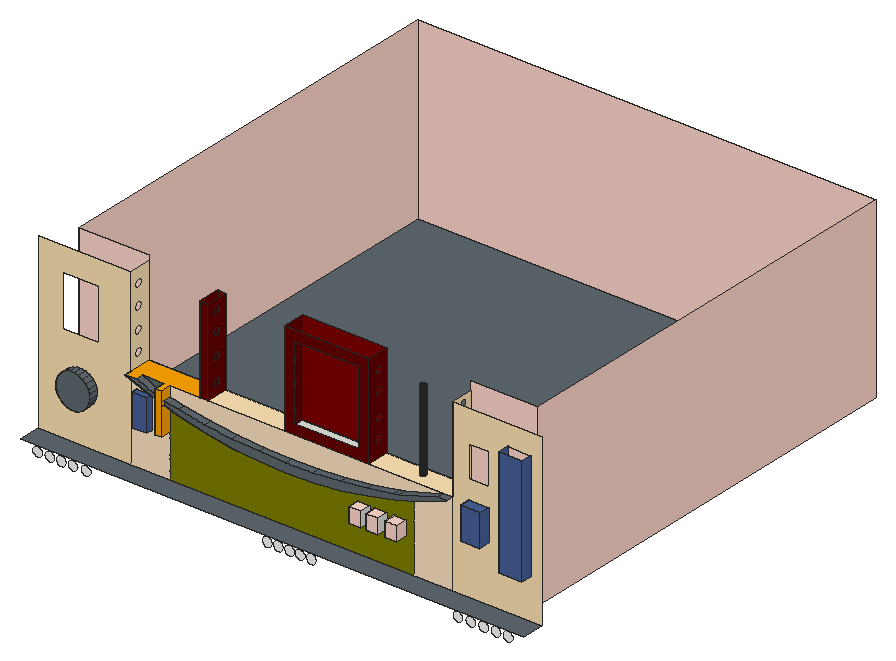
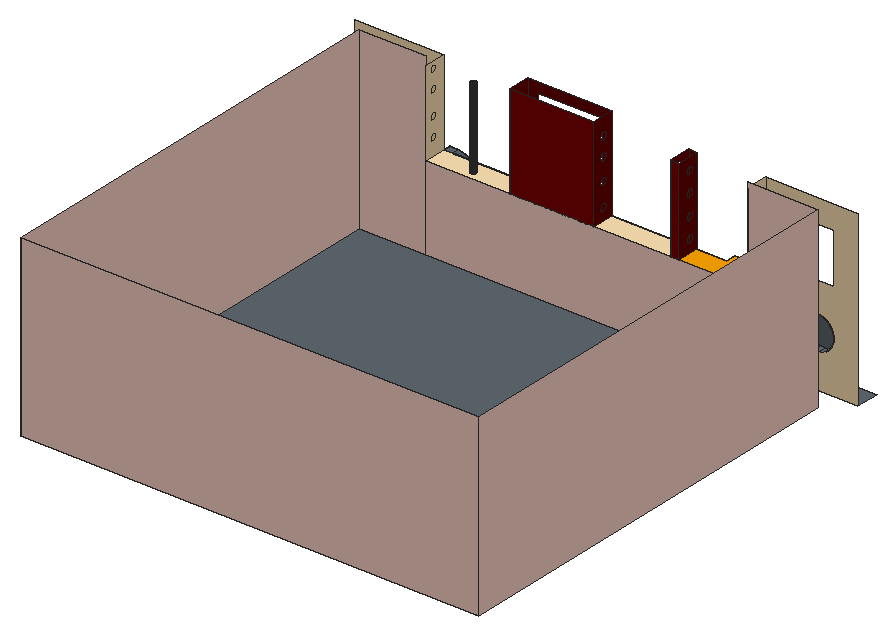
# SketchUp Ruby script. Lengths in inches.
U = 1.inch
M = Sketchup.active_model
def pt(a) = Geom::Point3d.new(a.map { |v| v * U })
def face(e, loops, mat)
  f = e.add_face(loops[0].map { |a| pt(a) })
  loops[1..].each { |l| e.add_face(l.map { |a| pt(a) }).erase! }
  f.material = f.back_material = mat if mat
  f
end
# faces: each face lists its corners as indices into pts; further lists are holes
def faces(e, pts, list, mat = nil) = list.each { |f| face(e, (f[0].is_a?(Array) ? f : [f]).map { |l| l.map { |i| pts[i] } }, mat) }
# xy, xz, yz: faces in a plane at the given z, y or x. An outline is a flat list of corners, or four numbers for a rectangle; further outlines are holes
def ring(l) = l.size == 4 ? [[l[0], l[1]], [l[2], l[1]], [l[2], l[3]], [l[0], l[3]]] : l.each_slice(2).to_a
def flat(e, list, mat, &to3) = list.each { |f| face(e, (f[0].is_a?(Array) ? f : [f]).map { |l| ring(l).map { |u, v| to3.(u, v) } }, mat) }
def xy(e, z, list, mat = nil) = flat(e, list, mat) { |x, y| [x, y, z] }
def xz(e, y, list, mat = nil) = flat(e, list, mat) { |x, z| [x, y, z] }
def yz(e, x, list, mat = nil) = flat(e, list, mat) { |y, z| [x, y, z] }
def lines(e, pts, list) = list.each { |a, b| e.add_line(pt(pts[a]), pt(pts[b])) }
# prism: a flat outline (further loops are holes) pulled along v
def prism(e, loops, v, mat = nil)
  f = face(e, loops, mat); d = Geom::Vector3d.new(v.map { |x| x * U })
  f.pushpull(f.normal.samedirection?(d) ? d.length : -d.length)
end
def box(e, o, s, mat = nil) = prism(e, [[o, [o[0] + s[0], o[1], o[2]], [o[0] + s[0], o[1] + s[1], o[2]], [o[0], o[1] + s[1], o[2]]]], [0, 0, s[2]], mat)
def at(x, y, z, deg = 0) = Geom::Transformation.translation(pt([x, y, z])) * Geom::Transformation.rotation(ORIGIN, Z_AXIS, deg.degrees)
def axes(o, x, y, z) = Geom::Transformation.new([*x, 0, *y, 0, *z, 0, *pt(o).to_a, 1])
def part(name) = M.definitions.add(name)
# library, detail: a bought-in or finely detailed component or shape, given as its bounding box
def library(name, o, s) = part(name).tap { |d| box(d.entities, o, s) }
def detail(e, o, s) = box(e.add_group.entities, o, s)
def put(e, d, t, mat = nil) = e.add_instance(d, t).tap { |i| i.material = mat if mat }
def group(e, t, mat = nil) = e.add_group.tap { |g| g.transformation = t; g.material = mat if mat }.entities
root = M.entities
M.materials.add("[0012_Bisque]").color = [255, 228, 196]
M.materials.add("[0022_Maroon]").color = [128, 0, 0]
M.materials.add("[0032_Moccasin]").color = [255, 228, 181]
M.materials.add("[0038_Orange]").color = [255, 165, 0]
M.materials.add("[0058_Olive]").color = [128, 128, 0]
M.materials.add("[Color A08]").color = [102, 0, 0]
M.materials.add("[Color B01]").color = [255, 216, 204]
M.materials.add("[Color M07]").color = [58, 58, 58]
M.materials.add("[Formica Blue]").color = [71, 97, 152]
M.materials.add("[Formica Speckled Grey]").color = [94, 105, 111]
M.materials.add("[Quartz Light Grey]").color = [251, 251, 252]
xy(root,133.625,[[47,20.01,251.02,29.17],[56.16,38.27,241.86,209.77]],"[Formica Speckled Grey]")
xy(root,146.7,[[176.27,24.54,181.08,29.17],[183.39,24.54,188.2,29.17],[191.08,24.54,195.89,29.17]],"[Color B01]")
xy(root,148.88,[[86.87,26.79,92.74,29.17]],"[Formica Blue]")
xy(root,149.75,[[236.96,24.73,246.46,29.17]],"[Formica Blue]")
xy(root,151.0625,[[97.68,24.86,100.35,29.17]],"[0038_Orange]")
xy(root,152.64,[[176.27,24.54,181.08,29.17],[183.39,24.54,188.2,29.17],[191.08,24.54,195.89,29.17]],"[Color B01]")
xy(root,155.96,[[221.42,24.73,229.42,29.17]],"[Formica Blue]")
xy(root,161.88,[[86.87,26.79,92.74,29.17]],"[Formica Blue]")
xy(root,167.625,[[112.25,29.17,115.75,38.27],[146.64,29.17,180.76,38.27]])
xy(root,167.625,[[115.75,29.17,146.64,38.27],[[180.76,29.17,214.88,38.27],[198.48,33.52,198.21,33.56,197.95,33.66,197.73,33.83,197.5625,34.05,197.46,34.31,197.42,34.58,197.46,34.86,197.5625,35.12,197.73,35.34,197.95,35.5,198.21,35.61,198.48,35.65,198.76,35.61,199.01,35.5,199.23,35.34,199.4,35.12,199.51,34.86,199.55,34.58,199.51,34.31,199.4,34.05,199.23,33.83,199.01,33.66,198.76,33.56]]],"[0032_Moccasin]")
xy(root,167.625,[[97.68,24.86,100.35,24.86,100.35,29.17,112.25,29.17,112.25,38.27,84.58,38.27,84.58,26.11,89.25,26.11,89.25,29.17,97.68,29.17]],"[0038_Orange]")
xy(root,167.625,[[211.24,26.11,214.88,29.17]],"[Formica Speckled Grey]")
xy(root,168.9,[[221.42,24.73,229.42,29.17]],"[Formica Blue]")
xz(root,20.01,[[54,129.67,54.47,129.73,54.9,129.91,55.28,130.2,55.57,130.57,55.75,131.01,55.81,131.48,55.75,131.95,55.57,132.38,55.28,132.76,54.9,133.05,54.47,133.23,54,133.29,53.53,133.23,53.09,133.05,52.72,132.76,52.43,132.38,52.25,131.95,52.19,131.48,52.25,131.01,52.43,130.57,52.72,130.2,53.09,129.91,53.53,129.73],[58.94,129.67,59.4,129.73,59.84,129.91,60.22,130.2,60.5,130.57,60.6875,131.01,60.75,131.48,60.6875,131.95,60.5,132.38,60.22,132.76,59.84,133.05,59.4,133.23,58.94,133.29,58.47,133.23,58.03,133.05,57.65,132.76,57.37,132.38,57.18,131.95,57.12,131.48,57.18,131.01,57.37,130.57,57.65,130.2,58.03,129.91,58.47,129.73],[63.56,129.67,64.03,129.73,64.47,129.91,64.84,130.2,65.13,130.57,65.3125,131.01,65.37,131.48,65.3125,131.95,65.13,132.38,64.84,132.76,64.47,133.05,64.03,133.23,63.56,133.29,63.09,133.23,62.65,133.05,62.28,132.76,61.99,132.38,61.81,131.95,61.75,131.48,61.81,131.01,61.99,130.57,62.28,130.2,62.65,129.91,63.09,129.73],[68.31,129.67,68.78,129.73,69.22,129.91,69.59,130.2,69.88,130.57,70.0625,131.01,70.12,131.48,70.0625,131.95,69.88,132.38,69.59,132.76,69.22,133.05,68.78,133.23,68.31,133.29,67.84,133.23,67.4,133.05,67.03,132.76,66.74,132.38,66.56,131.95,66.5,131.48,66.56,131.01,66.74,130.57,67.03,130.2,67.4,129.91,67.84,129.73],[73.62,129.67,74.09,129.73,74.53,129.91,74.9,130.2,75.19,130.57,75.375,131.01,75.44,131.48,75.375,131.95,75.19,132.38,74.9,132.76,74.53,133.05,74.09,133.23,73.62,133.29,73.15,133.23,72.72,133.05,72.34,132.76,72.05,132.38,71.87,131.95,71.81,131.48,71.87,131.01,72.05,130.57,72.34,130.2,72.72,129.91,73.15,129.73],
  [147.06,129.67,147.53,129.73,147.97,129.91,148.34,130.2,148.63,130.57,148.8125,131.01,148.87,131.48,148.8125,131.95,148.63,132.38,148.34,132.76,147.97,133.05,147.53,133.23,147.06,133.29,146.59,133.23,146.15,133.05,145.78,132.76,145.49,132.38,145.31,131.95,145.25,131.48,145.31,131.01,145.49,130.57,145.78,130.2,146.15,129.91,146.59,129.73],[151.44,129.67,151.9,129.73,152.34,129.91,152.72,130.2,153,130.57,153.1875,131.01,153.25,131.48,153.1875,131.95,153,132.38,152.72,132.76,152.34,133.05,151.9,133.23,151.44,133.29,150.97,133.23,150.53,133.05,150.15,132.76,149.87,132.38,149.68,131.95,149.62,131.48,149.68,131.01,149.87,130.57,150.15,130.2,150.53,129.91,150.97,129.73],[156,129.67,156.47,129.73,156.9,129.91,157.28,130.2,157.57,130.57,157.75,131.01,157.81,131.48,157.75,131.95,157.57,132.38,157.28,132.76,156.9,133.05,156.47,133.23,156,133.29,155.53,133.23,155.09,133.05,154.72,132.76,154.43,132.38,154.25,131.95,154.19,131.48,154.25,131.01,154.43,130.57,154.72,130.2,155.09,129.91,155.53,129.73],[160.31,129.67,160.78,129.73,161.22,129.91,161.59,130.2,161.88,130.57,162.0625,131.01,162.12,131.48,162.0625,131.95,161.88,132.38,161.59,132.76,161.22,133.05,160.78,133.23,160.31,133.29,159.84,133.23,159.4,133.05,159.03,132.76,158.74,132.38,158.56,131.95,158.5,131.48,158.56,131.01,158.74,130.57,159.03,130.2,159.4,129.91,159.84,129.73],[164.87,129.67,165.34,129.73,165.78,129.91,166.15,130.2,166.44,130.57,166.625,131.01,166.69,131.48,166.625,131.95,166.44,132.38,166.15,132.76,165.78,133.05,165.34,133.23,164.87,133.29,164.4,133.23,163.97,133.05,163.59,132.76,163.3,132.38,163.12,131.95,163.06,131.48,163.12,131.01,163.3,130.57,163.59,130.2,163.97,129.91,164.4,129.73],
  [224.19,129.67,224.65,129.73,225.09,129.91,225.47,130.2,225.75,130.57,225.9375,131.01,226,131.48,225.9375,131.95,225.75,132.38,225.47,132.76,225.09,133.05,224.65,133.23,224.19,133.29,223.72,133.23,223.28,133.05,222.9,132.76,222.62,132.38,222.43,131.95,222.37,131.48,222.43,131.01,222.62,130.57,222.9,130.2,223.28,129.91,223.72,129.73],[229.44,129.67,229.9,129.73,230.34,129.91,230.72,130.2,231,130.57,231.1875,131.01,231.25,131.48,231.1875,131.95,231,132.38,230.72,132.76,230.34,133.05,229.9,133.23,229.44,133.29,228.97,133.23,228.53,133.05,228.15,132.76,227.87,132.38,227.68,131.95,227.62,131.48,227.68,131.01,227.87,130.57,228.15,130.2,228.53,129.91,228.97,129.73],[234.56,129.67,235.03,129.73,235.47,129.91,235.84,130.2,236.13,130.57,236.3125,131.01,236.37,131.48,236.3125,131.95,236.13,132.38,235.84,132.76,235.47,133.05,235.03,133.23,234.56,133.29,234.09,133.23,233.65,133.05,233.28,132.76,232.99,132.38,232.81,131.95,232.75,131.48,232.81,131.01,232.99,130.57,233.28,130.2,233.65,129.91,234.09,129.73],[239.62,129.67,240.09,129.73,240.53,129.91,240.9,130.2,241.19,130.57,241.375,131.01,241.44,131.48,241.375,131.95,241.19,132.38,240.9,132.76,240.53,133.05,240.09,133.23,239.62,133.29,239.15,133.23,238.72,133.05,238.34,132.76,238.05,132.38,237.87,131.95,237.81,131.48,237.87,131.01,238.05,130.57,238.34,130.2,238.72,129.91,239.15,129.73],[244.56,129.67,245.03,129.73,245.47,129.91,245.84,130.2,246.13,130.57,246.3125,131.01,246.37,131.48,246.3125,131.95,246.13,132.38,245.84,132.76,245.47,133.05,245.03,133.23,244.56,133.29,244.09,133.23,243.65,133.05,243.28,132.76,242.99,132.38,242.81,131.95,242.75,131.48,242.81,131.01,242.99,130.57,243.28,130.2,243.65,129.91,244.09,129.73]],"[Quartz Light Grey]")
xz(root,24.54,[[176.27,146.7,181.08,152.64],[183.39,146.7,188.2,152.64],[191.08,146.7,195.89,152.64]],"[Color B01]")
xz(root,24.73,[[236.96,149.75,246.46,193.75],[221.42,155.96,229.42,168.9]],"[Formica Blue]")
xz(root,24.86,[[97.68,151.0625,100.35,167.625]],"[0038_Orange]")
xz(root,25.54,[[63.21,147.56,65.04,147.63,66.78,148.17,68.33,149.14,69.57,150.48,70.42,152.1,70.83,153.88,70.76,155.7,70.22,157.45,69.25,159,67.91,160.24,66.29,161.09,64.51,161.5,62.68,161.43,60.9375,160.89,59.39,159.92,58.15,158.57,57.29,156.96,56.89,155.18,56.96,153.35,57.5,151.61,58.47,150.06,59.8125,148.82,61.43,147.96]],"[Formica Speckled Grey]")
xz(root,26.11,[[149.73,154.76,160.86,155.12,171.95,156.2,182.9375,158,193.79,160.52,199.12,162.12,204.45,163.73,214.88,167.625,211.24,167.625,195.42,163.01,193.47,162.6,182.62,160.83,171.7,159.57,160.73,158.81,149.73,158.55,138.74,158.81,127.77,159.57,116.84,160.83,105.99,162.6,100.35,163.79,100.35,162.12,105.68,160.52,116.53,158,127.52,156.2,138.6,155.12],[97.68,162.92,97.68,164.35,96.14,164.67,89.25,167.625,84.58,167.625,95.02,163.73]],"[Formica Speckled Grey]")
xz(root,26.79,[[86.87,148.88,92.74,161.88]],"[Formica Blue]")
xz(root,29.17,[[[84.58,133.625,100.35,133.625,100.35,151.0625,97.68,151.0625,97.68,162.92,95.02,163.73,84.58,167.625],[86.87,148.88,92.74,161.88]],[199.12,133.625,214.88,133.625,214.88,167.625,204.45,163.73,199.12,162.12],[149.73,158.55,160.73,158.81,171.7,159.57,182.62,160.83,193.47,162.6,195.42,163.01,211.24,167.625,100.35,167.625,100.35,163.79,105.99,162.6,116.84,160.83,127.77,159.57,138.74,158.81]],"[0012_Bisque]")
xz(root,29.17,[[[47,133.625,84.58,203.49],[56.92,173.26,71.36,193.95],[63.21,147.56,61.43,147.96,59.8125,148.82,58.47,150.06,57.5,151.61,56.96,153.35,56.89,155.18,57.29,156.96,58.15,158.57,59.39,159.92,60.9375,160.89,62.68,161.43,64.51,161.5,66.29,161.09,67.91,160.24,69.25,159,70.22,157.45,70.76,155.7,70.83,153.88,70.42,152.1,69.57,150.48,68.33,149.14,66.78,148.17,65.04,147.63]],[[214.88,133.625,251.02,202.04],[236.96,149.75,246.46,193.75],[221.42,176.39,229.42,189.34],[221.42,155.96,229.42,168.9]]],"[0032_Moccasin]")
xz(root,29.17,[[[100.35,133.625,199.12,133.625,199.12,162.12,193.79,160.52,182.9375,158,171.95,156.2,160.86,155.12,149.73,154.76,138.6,155.12,127.52,156.2,116.53,158,105.68,160.52,100.35,162.12],[191.08,146.7,195.89,152.64],[183.39,146.7,188.2,152.64],[176.27,146.7,181.08,152.64]]],"[0058_Olive]")
xz(root,29.17,[[112.25,167.625,115.75,202.625],[[146.64,167.625,180.76,205.625],[150.55,171.54,176.84,201.71]]],"[Color A08]")
xz(root,29.17,[[97.68,164.35,97.68,167.625,89.25,167.625,96.14,164.67]],"[Formica Speckled Grey]")
xz(root,38.27,[[112.25,167.625,115.75,202.625],[146.64,167.625,180.76,205.625]],"[0022_Maroon]")
xz(root,38.27,[[56.16,133.625,84.58,205.625],[84.58,133.625,214.88,167.625],[214.88,133.625,241.86,205.625]],"[Color B01]")
xz(root,209.77,[[56.16,133.625,241.86,205.625]],"[Color B01]")
yz(root,56.16,[[38.27,133.625,209.77,205.625]],"[Color B01]")
yz(root,84.58,[[[29.17,167.625,38.27,203.49],[32.81,171.26,32.39,171.3125,32,171.47,31.66,171.73,31.4,172.07,31.24,172.46,31.18,172.88,31.24,173.3,31.4,173.69,31.66,174.03,32,174.29,32.39,174.45,32.81,174.51,33.23,174.45,33.62,174.29,33.96,174.03,34.22,173.69,34.38,173.3,34.43,172.88,34.38,172.46,34.22,172.07,33.96,171.73,33.62,171.47,33.23,171.3125],[32.81,179.38,32.39,179.4375,32,179.6,31.66,179.86,31.4,180.19,31.24,180.59,31.18,181.01,31.24,181.43,31.4,181.82,31.66,182.16,32,182.41,32.39,182.58,32.81,182.63,33.23,182.58,33.62,182.41,33.96,182.16,34.22,181.82,34.38,181.43,34.43,181.01,34.38,180.59,34.22,180.19,33.96,179.86,33.62,179.6,33.23,179.4375],[32.81,188.01,32.39,188.0625,32,188.22,31.66,188.48,31.4,188.82,31.24,189.21,31.18,189.63,31.24,190.05,31.4,190.44,31.66,190.78,32,191.04,32.39,191.2,32.81,191.26,33.23,191.2,33.62,191.04,33.96,190.78,34.22,190.44,34.38,190.05,34.43,189.63,34.38,189.21,34.22,188.82,33.96,188.48,33.62,188.22,33.23,188.0625],[32.81,196.19,32.39,196.25,32,196.41,31.66,196.67,31.4,197.01,31.24,197.4,31.18,197.82,31.24,198.24,31.4,198.63,31.66,198.97,32,199.23,32.39,199.39,32.81,199.44,33.23,199.39,33.62,199.23,33.96,198.97,34.22,198.63,34.38,198.24,34.43,197.82,34.38,197.4,34.22,197.01,33.96,196.67,33.62,196.41,33.23,196.25]]],"[0032_Moccasin]")
yz(root,86.87,[[26.79,148.88,29.17,161.88]],"[Formica Blue]")
yz(root,92.74,[[26.79,148.88,29.17,161.88]],"[Formica Blue]")
yz(root,97.68,[[24.86,151.0625,29.17,162.92],[24.86,162.92,26.11,164.35],[24.86,164.35,29.17,167.625]],"[0038_Orange]")
yz(root,100.35,[[24.86,151.0625,29.17,162.12],[24.86,162.12,26.11,163.79],[24.86,163.79,29.17,167.625]],"[0038_Orange]")
yz(root,112.25,[[[29.17,167.625,38.27,202.625],[32.81,196.19,33.23,196.25,33.62,196.41,33.96,196.67,34.22,197.01,34.38,197.4,34.43,197.82,34.38,198.24,34.22,198.63,33.96,198.97,33.62,199.23,33.23,199.39,32.81,199.44,32.39,199.39,32,199.23,31.66,198.97,31.4,198.63,31.24,198.24,31.18,197.82,31.24,197.4,31.4,197.01,31.66,196.67,32,196.41,32.39,196.25],[32.81,171.26,33.23,171.3125,33.62,171.47,33.96,171.73,34.22,172.07,34.38,172.46,34.43,172.88,34.38,173.3,34.22,173.69,33.96,174.03,33.62,174.29,33.23,174.45,32.81,174.51,32.39,174.45,32,174.29,31.66,174.03,31.4,173.69,31.24,173.3,31.18,172.88,31.24,172.46,31.4,172.07,31.66,171.73,32,171.47,32.39,171.3125],[32.81,188.01,33.23,188.0625,33.62,188.22,33.96,188.48,34.22,188.82,34.38,189.21,34.43,189.63,34.38,190.05,34.22,190.44,33.96,190.78,33.62,191.04,33.23,191.2,32.81,191.26,32.39,191.2,32,191.04,31.66,190.78,31.4,190.44,31.24,190.05,31.18,189.63,31.24,189.21,31.4,188.82,31.66,188.48,32,188.22,32.39,188.0625],[32.81,179.38,33.23,179.4375,33.62,179.6,33.96,179.86,34.22,180.19,34.38,180.59,34.43,181.01,34.38,181.43,34.22,181.82,33.96,182.16,33.62,182.41,33.23,182.58,32.81,182.63,32.39,182.58,32,182.41,31.66,182.16,31.4,181.82,31.24,181.43,31.18,181.01,31.24,180.59,31.4,180.19,31.66,179.86,32,179.6,32.39,179.4375]]],"[Color A08]")
yz(root,115.75,[[[29.17,167.625,38.27,202.625],[33.57,196.94,33.15,197,32.76,197.16,32.42,197.42,32.17,197.76,32,198.15,31.95,198.57,32,198.99,32.17,199.38,32.42,199.72,32.76,199.98,33.15,200.14,33.57,200.19,33.99,200.14,34.39,199.98,34.72,199.72,34.98,199.38,35.14,198.99,35.2,198.57,35.14,198.15,34.98,197.76,34.72,197.42,34.39,197.16,33.99,197],[33.57,170.94,33.15,171,32.76,171.16,32.42,171.42,32.17,171.76,32,172.15,31.95,172.57,32,172.99,32.17,173.38,32.42,173.72,32.76,173.98,33.15,174.14,33.57,174.19,33.99,174.14,34.39,173.98,34.72,173.72,34.98,173.38,35.14,172.99,35.2,172.57,35.14,172.15,34.98,171.76,34.72,171.42,34.39,171.16,33.99,171],[33.57,189.26,33.15,189.3125,32.76,189.47,32.42,189.73,32.17,190.07,32,190.46,31.95,190.88,32,191.3,32.17,191.69,32.42,192.03,32.76,192.29,33.15,192.45,33.57,192.51,33.99,192.45,34.39,192.29,34.72,192.03,34.98,191.69,35.14,191.3,35.2,190.88,35.14,190.46,34.98,190.07,34.72,189.73,34.39,189.47,33.99,189.3125],[33.57,180.44,33.15,180.5,32.76,180.66,32.42,180.92,32.17,181.26,32,181.65,31.95,182.07,32,182.49,32.17,182.88,32.42,183.22,32.76,183.48,33.15,183.64,33.57,183.69,33.99,183.64,34.39,183.48,34.72,183.22,34.98,182.88,35.14,182.49,35.2,182.07,35.14,181.65,34.98,181.26,34.72,180.92,34.39,180.66,33.99,180.5]]],"[Color A08]")
yz(root,146.64,[[[29.17,167.625,38.27,205.625],[33.57,196.94,33.99,197,34.39,197.16,34.72,197.42,34.98,197.76,35.14,198.15,35.2,198.57,35.14,198.99,34.98,199.38,34.72,199.72,34.39,199.98,33.99,200.14,33.57,200.19,33.15,200.14,32.76,199.98,32.42,199.72,32.17,199.38,32,198.99,31.95,198.57,32,198.15,32.17,197.76,32.42,197.42,32.76,197.16,33.15,197],[33.57,189.26,33.99,189.3125,34.39,189.47,34.72,189.73,34.98,190.07,35.14,190.46,35.2,190.88,35.14,191.3,34.98,191.69,34.72,192.03,34.39,192.29,33.99,192.45,33.57,192.51,33.15,192.45,32.76,192.29,32.42,192.03,32.17,191.69,32,191.3,31.95,190.88,32,190.46,32.17,190.07,32.42,189.73,32.76,189.47,33.15,189.3125],[33.57,180.44,33.99,180.5,34.39,180.66,34.72,180.92,34.98,181.26,35.14,181.65,35.2,182.07,35.14,182.49,34.98,182.88,34.72,183.22,34.39,183.48,33.99,183.64,33.57,183.69,33.15,183.64,32.76,183.48,32.42,183.22,32.17,182.88,32,182.49,31.95,182.07,32,181.65,32.17,181.26,32.42,180.92,32.76,180.66,33.15,180.5],[33.57,170.94,33.99,171,34.39,171.16,34.72,171.42,34.98,171.76,35.14,172.15,35.2,172.57,35.14,172.99,34.98,173.38,34.72,173.72,34.39,173.98,33.99,174.14,33.57,174.19,33.15,174.14,32.76,173.98,32.42,173.72,32.17,173.38,32,172.99,31.95,172.57,32,172.15,32.17,171.76,32.42,171.42,32.76,171.16,33.15,171]]],"[Color A08]")
yz(root,176.27,[[24.54,146.7,29.17,152.64]],"[Color B01]")
yz(root,180.76,[[[29.17,167.625,38.27,205.625],[34.44,197.93,34.07,197.96,33.71,198.09,33.41,198.31,33.17,198.59,33.01,198.94,32.95,199.31,32.98,199.68,33.11,200.03,33.33,200.34,33.62,200.58,33.96,200.73,34.33,200.8,34.7,200.76,35.05,200.63,35.36,200.42,35.6,200.13,35.76,199.79,35.82,199.42,35.79,199.05,35.66,198.69,35.4375,198.39,35.15,198.15,34.81,197.99],[34.44,190.43,34.07,190.46,33.71,190.59,33.41,190.81,33.17,191.09,33.01,191.44,32.95,191.81,32.98,192.18,33.11,192.53,33.33,192.84,33.62,193.08,33.96,193.23,34.33,193.3,34.7,193.26,35.05,193.13,35.36,192.92,35.6,192.63,35.76,192.29,35.82,191.92,35.79,191.55,35.66,191.19,35.4375,190.89,35.15,190.65,34.81,190.49],[34.44,180.68,34.07,180.71,33.71,180.84,33.41,181.06,33.17,181.34,33.01,181.69,32.95,182.06,32.98,182.43,33.11,182.78,33.33,183.09,33.62,183.33,33.96,183.48,34.33,183.55,34.7,183.51,35.05,183.38,35.36,183.17,35.6,182.88,35.76,182.54,35.82,182.17,35.79,181.8,35.66,181.44,35.4375,181.14,35.15,180.9,34.81,180.74],[34.44,173.05,34.07,173.08,33.71,173.21,33.41,173.43,33.17,173.72,33.01,174.06,32.95,174.43,32.98,174.8,33.11,175.16,33.33,175.46,33.62,175.7,33.96,175.86,34.33,175.92,34.7,175.89,35.05,175.76,35.36,175.54,35.6,175.25,35.76,174.91,35.82,174.54,35.79,174.17,35.66,173.82,35.4375,173.51,35.15,173.27,34.81,173.11]]],"[Color A08]")
yz(root,181.08,[[24.54,146.7,29.17,152.64]])
yz(root,183.39,[[24.54,146.7,29.17,152.64]],"[Color B01]")
yz(root,188.2,[[24.54,146.7,29.17,152.64]])
yz(root,191.08,[[24.54,146.7,29.17,152.64]],"[Color B01]")
yz(root,195.89,[[24.54,146.7,29.17,152.64]],"[Color B01]")
yz(root,214.88,[[[29.17,167.625,38.27,202.04],[34.44,197.93,34.81,197.99,35.15,198.15,35.4375,198.39,35.66,198.69,35.79,199.05,35.82,199.42,35.76,199.79,35.6,200.13,35.36,200.42,35.05,200.63,34.7,200.76,34.33,200.8,33.96,200.73,33.62,200.58,33.33,200.34,33.11,200.03,32.98,199.68,32.95,199.31,33.01,198.94,33.17,198.59,33.41,198.31,33.71,198.09,34.07,197.96],[34.44,173.05,34.81,173.11,35.15,173.27,35.4375,173.51,35.66,173.82,35.79,174.17,35.82,174.54,35.76,174.91,35.6,175.25,35.36,175.54,35.05,175.76,34.7,175.89,34.33,175.92,33.96,175.86,33.62,175.7,33.33,175.46,33.11,175.16,32.98,174.8,32.95,174.43,33.01,174.06,33.17,173.72,33.41,173.43,33.71,173.21,34.07,173.08],[34.44,190.43,34.81,190.49,35.15,190.65,35.4375,190.89,35.66,191.19,35.79,191.55,35.82,191.92,35.76,192.29,35.6,192.63,35.36,192.92,35.05,193.13,34.7,193.26,34.33,193.3,33.96,193.23,33.62,193.08,33.33,192.84,33.11,192.53,32.98,192.18,32.95,191.81,33.01,191.44,33.17,191.09,33.41,190.81,33.71,190.59,34.07,190.46],[34.44,180.68,34.81,180.74,35.15,180.9,35.4375,181.14,35.66,181.44,35.79,181.8,35.82,182.17,35.76,182.54,35.6,182.88,35.36,183.17,35.05,183.38,34.7,183.51,34.33,183.55,33.96,183.48,33.62,183.33,33.33,183.09,33.11,182.78,32.98,182.43,32.95,182.06,33.01,181.69,33.17,181.34,33.41,181.06,33.71,180.84,34.07,180.71]]],"[0032_Moccasin]")
yz(root,221.42,[[24.73,155.96,29.17,168.9]],"[Formica Blue]")
yz(root,229.42,[[24.73,155.96,29.17,168.9]],"[Formica Blue]")
yz(root,236.96,[[24.73,149.75,29.17,193.75]],"[Formica Blue]")
yz(root,241.86,[[38.27,133.625,209.77,205.625]],"[Color B01]")
yz(root,246.46,[[24.73,149.75,29.17,193.75]],"[Formica Blue]")
p = [[61.43,29.17,147.96],[63.21,29.17,147.56],[63.21,25.54,147.56],[61.43,25.54,147.96],[65.04,29.17,147.63],[65.04,25.54,147.63],
  [66.78,29.17,148.17],[66.78,25.54,148.17],[59.8125,29.17,148.82],[59.8125,25.54,148.82],[68.33,29.17,149.14],[68.33,25.54,149.14],
  [58.47,29.17,150.06],[58.47,25.54,150.06],[69.57,29.17,150.48],[69.57,25.54,150.48],[57.5,29.17,151.61],[57.5,25.54,151.61],
  [70.42,29.17,152.1],[70.42,25.54,152.1],[56.96,29.17,153.35],[56.96,25.54,153.35],[70.83,29.17,153.88],[70.83,25.54,153.88],
  [56.89,29.17,155.18],[56.89,25.54,155.18],[70.76,29.17,155.7],[70.76,25.54,155.7],[138.6,29.17,155.12],[149.73,29.17,154.76],
  [149.73,26.11,154.76],[138.6,26.11,155.12],[160.86,29.17,155.12],[160.86,26.11,155.12],[127.52,29.17,156.2],[127.52,26.11,156.2],
  [171.95,29.17,156.2],[171.95,26.11,156.2],[57.29,29.17,156.96],[57.29,25.54,156.96],[70.22,29.17,157.45],[70.22,25.54,157.45],
  [116.53,29.17,158],[116.53,26.11,158],[182.9375,29.17,158],[182.9375,26.11,158],[58.15,29.17,158.57],[58.15,25.54,158.57],
  [69.25,29.17,159],[69.25,25.54,159],[105.68,29.17,160.52],[105.68,26.11,160.52],[193.79,29.17,160.52],[193.79,26.11,160.52],
  [59.39,29.17,159.92],[59.39,25.54,159.92],[149.73,29.17,158.55],[138.74,29.17,158.81],[138.74,26.11,158.81],[149.73,26.11,158.55],
  [160.73,29.17,158.81],[160.73,26.11,158.81],[127.77,29.17,159.57],[127.77,26.11,159.57],[171.7,29.17,159.57],[171.7,26.11,159.57],
  [67.91,29.17,160.24],[67.91,25.54,160.24],[116.84,29.17,160.83],[116.84,26.11,160.83],[182.62,29.17,160.83],[182.62,26.11,160.83],
  [60.9375,29.17,160.89],[60.9375,25.54,160.89],[66.29,29.17,161.09],[66.29,25.54,161.09],[100.35,29.17,162.12],[100.35,26.11,162.12],
  [199.12,29.17,162.12],[199.12,26.11,162.12],[105.99,29.17,162.6],[105.99,26.11,162.6],[193.47,29.17,162.6],[193.47,26.11,162.6],
  [62.68,29.17,161.43],[62.68,25.54,161.43],[64.51,29.17,161.5],[64.51,25.54,161.5],[204.45,29.17,163.73],[204.45,26.11,163.73],
  [100.35,29.17,163.79],[100.35,26.11,163.79],[195.42,29.17,163.01],[195.42,26.11,163.01],[95.02,29.17,163.73],[97.68,29.17,162.92],
  [97.68,26.11,162.92],[95.02,26.11,163.73],[211.24,29.17,167.625],[211.24,26.11,167.625],[84.58,29.17,167.625],[84.58,26.11,167.625],
  [214.88,29.17,167.625],[214.88,26.11,167.625],[97.68,29.17,164.35],[96.14,29.17,164.67],[96.14,26.11,164.67],[97.68,26.11,164.35],
  [89.25,29.17,167.625],[89.25,26.11,167.625],[198.21,33.56,167.625],[198.48,33.52,167.625],[198.48,33.52,200.34],[198.21,33.56,200.34],
  [198.76,33.56,167.625],[198.76,33.56,200.34],[197.95,33.66,167.625],[197.95,33.66,200.34],[199.01,33.66,167.625],[199.01,33.66,200.34],
  [197.73,33.83,167.625],[197.73,33.83,200.34],[199.23,33.83,167.625],[199.23,33.83,200.34],[197.5625,34.05,167.625],[197.5625,34.05,200.34],
  [199.4,34.05,167.625],[199.4,34.05,200.34],[197.46,34.31,167.625],[197.46,34.31,200.34],[199.51,34.31,167.625],[199.51,34.31,200.34],
  [197.42,34.58,167.625],[197.42,34.58,200.34],[199.55,34.58,167.625],[199.55,34.58,200.34],[197.46,34.86,167.625],[197.46,34.86,200.34],
  [199.51,34.86,167.625],[199.51,34.86,200.34],[197.5625,35.12,167.625],[197.5625,35.12,200.34],[199.4,35.12,167.625],[199.4,35.12,200.34],
  [197.73,35.34,167.625],[197.73,35.34,200.34],[199.23,35.34,167.625],[199.23,35.34,200.34],[197.95,35.5,167.625],[197.95,35.5,200.34],
  [199.01,35.5,167.625],[199.01,35.5,200.34],[198.21,35.61,167.625],[198.21,35.61,200.34],[198.76,35.61,167.625],[198.76,35.61,200.34],
  [198.48,35.65,167.625],[198.48,35.65,200.34]]
faces(root,p,[[0,1,2,3],[1,4,5,2],[4,6,7,5],[8,0,3,9],[6,10,11,7],[12,8,9,13],[10,14,15,11],[16,12,13,17],
  [14,18,19,15],[20,16,17,21],[18,22,23,19],[24,20,21,25],[22,26,27,23],[28,29,30,31],[29,32,33,30],[34,28,31,35],
  [32,36,37,33],[38,24,25,39],[26,40,41,27],[42,34,35,43],[36,44,45,37],[46,38,39,47],[40,48,49,41],[50,42,43,51],
  [44,52,53,45],[54,46,47,55],[56,57,58,59],[60,56,59,61],[57,62,63,58],[64,60,61,65],[48,66,67,49],[62,68,69,63],
  [70,64,65,71],[72,54,55,73],[66,74,75,67],[76,50,51,77],[52,78,79,53],[68,80,81,69],[82,70,71,83],[84,72,73,85],
  [74,86,87,75],[86,84,85,87],[78,88,89,79],[80,90,91,81],[92,82,83,93],[94,95,96,97],[98,92,93,99],[100,94,97,101],
  [88,102,103,89],[104,105,106,107],[105,108,109,106]],"[Formica Speckled Grey]")
faces(root,p,[[110,111,112,113],[111,114,115,112],[116,110,113,117],[114,118,119,115],[120,116,117,121],[118,122,123,119],[124,120,121,125],[122,126,127,123],
  [128,124,125,129],[126,130,131,127],[132,128,129,133],[130,134,135,131],[136,132,133,137],[134,138,139,135],[140,136,137,141],[138,142,143,139],
  [144,140,141,145],[142,146,147,143],[148,144,145,149],[146,150,151,147],[152,148,149,153],[150,154,155,151],[156,152,153,157],[154,156,157,155]],"[Color M07]")
